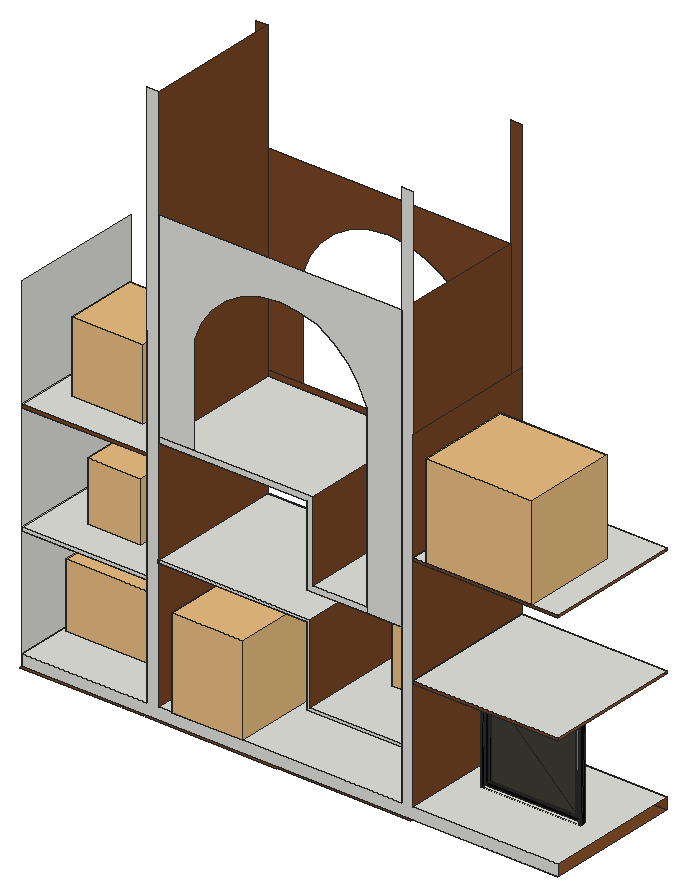
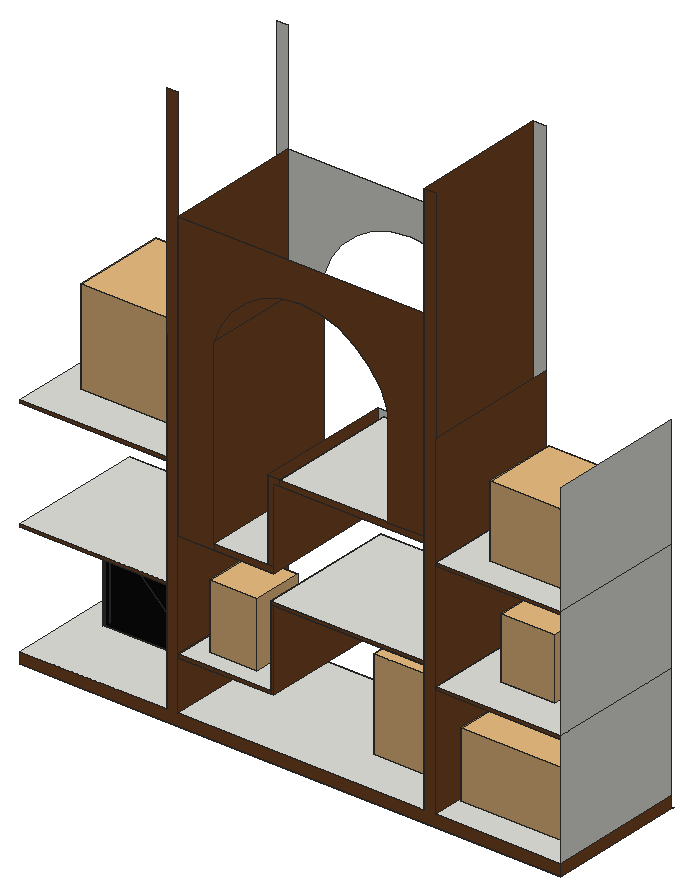
# SketchUp Ruby script. Lengths in inches.
U = 1.inch
M = Sketchup.active_model
def pt(a) = Geom::Point3d.new(a.map { |v| v * U })
def face(e, loops, mat)
  f = e.add_face(loops[0].map { |a| pt(a) })
  loops[1..].each { |l| e.add_face(l.map { |a| pt(a) }).erase! }
  f.material = f.back_material = mat if mat
  f
end
# faces: each face lists its corners as indices into pts; further lists are holes
def faces(e, pts, list, mat = nil) = list.each { |f| face(e, (f[0].is_a?(Array) ? f : [f]).map { |l| l.map { |i| pts[i] } }, mat) }
# xy, xz, yz: faces in a plane at the given z, y or x. An outline is a flat list of corners, or four numbers for a rectangle; further outlines are holes
def ring(l) = l.size == 4 ? [[l[0], l[1]], [l[2], l[1]], [l[2], l[3]], [l[0], l[3]]] : l.each_slice(2).to_a
def flat(e, list, mat, &to3) = list.each { |f| face(e, (f[0].is_a?(Array) ? f : [f]).map { |l| ring(l).map { |u, v| to3.(u, v) } }, mat) }
def xy(e, z, list, mat = nil) = flat(e, list, mat) { |x, y| [x, y, z] }
def xz(e, y, list, mat = nil) = flat(e, list, mat) { |x, z| [x, y, z] }
def yz(e, x, list, mat = nil) = flat(e, list, mat) { |y, z| [x, y, z] }
def lines(e, pts, list) = list.each { |a, b| e.add_line(pt(pts[a]), pt(pts[b])) }
# prism: a flat outline (further loops are holes) pulled along v
def prism(e, loops, v, mat = nil)
  f = face(e, loops, mat); d = Geom::Vector3d.new(v.map { |x| x * U })
  f.pushpull(f.normal.samedirection?(d) ? d.length : -d.length)
end
def box(e, o, s, mat = nil) = prism(e, [[o, [o[0] + s[0], o[1], o[2]], [o[0] + s[0], o[1] + s[1], o[2]], [o[0], o[1] + s[1], o[2]]]], [0, 0, s[2]], mat)
def at(x, y, z, deg = 0) = Geom::Transformation.translation(pt([x, y, z])) * Geom::Transformation.rotation(ORIGIN, Z_AXIS, deg.degrees)
def axes(o, x, y, z) = Geom::Transformation.new([*x, 0, *y, 0, *z, 0, *pt(o).to_a, 1])
def part(name) = M.definitions.add(name)
# library, detail: a bought-in or finely detailed component or shape, given as its bounding box
def library(name, o, s) = part(name).tap { |d| box(d.entities, o, s) }
def detail(e, o, s) = box(e.add_group.entities, o, s)
def put(e, d, t, mat = nil) = e.add_instance(d, t).tap { |i| i.material = mat if mat }
def group(e, t, mat = nil) = e.add_group.tap { |g| g.transformation = t; g.material = mat if mat }.entities
root = M.entities
M.materials.add("Material~12").color = [12, 12, 12]
M.materials.add("Material~27").color = [10, 10, 10]
M.materials.add("Material~28").color = [156, 145, 125]
M.materials.add("Material~29").color = [62, 62, 54]
M.materials.add("[Wood Veneer 01]").color = [120, 70, 37]
c1 = library("Group3\#1",[-226.43,63.68,0],[21.09,21.08,29.58])
c2 = library("Group145\#1",[5.875,6.46,9.56],[20.8,10.13,11.36])
c3 = library("Potted Plant",[38.42,1.35,0],[44.68,49.99,41.74])
c4 = library("Pot Nice",[-24.73,-24.73,-0.79],[49.46,49.46,53.07])
c5 = library("Desktop globe",[0,0,0],[12.93,11.94,21.27])
c6 = library("PLANTS",[8.46,16.75,1.64],[23.16,16.42,22.13])
c7 = part("3DGeom~7_Defintion")
xy(c7.entities,14.63,[[-469.76,-662.07,-453.03,-645.34,-469.55,277.5],[-469.76,-662.07,513.32,-645.34,-453.03,-645.34],[-469.76,-662.07,530.04,-662.07,513.32,-645.34],[530.04,-662.07,513.52,260.77,513.32,-645.34],[530.04,-662.07,530.24,277.5,513.52,260.77],
  [-453.03,-645.34,-452.83,260.77,-469.55,277.5],[-452.83,260.77,530.24,277.5,-469.55,277.5],[-452.83,260.77,513.52,260.77,530.24,277.5]])
xz(c7.entities,-645.34,[[-453.03,2.4375,-453.03,14.63,513.32,2.4375],[513.32,2.4375,-453.03,14.63,513.32,14.63]])
xz(c7.entities,260.77,[[-452.83,2.4375,513.52,14.63,-452.83,14.63],[-452.83,2.4375,513.52,2.4375,513.52,14.63]])
p = [[-452.83,260.77,14.63],[-453.03,-645.34,14.63],[-453.03,-645.34,2.4375],[-452.83,260.77,2.4375],[513.32,-645.34,14.63],[513.52,260.77,14.63],
  [513.52,260.77,2.4375],[513.32,-645.34,2.4375]]
faces(c7.entities,p,[[0,1,2],[2,3,0],[4,5,6],[6,7,4]])
c8 = part("Group74\#2")
put(c8.entities,c7,axes([-1.26,-0.81,45.42],[0.01556,0,0],[0,0,0.01556],[0,-0.0137,0]),"Material~27")
c9 = part("Group73\#2")
put(c9.entities,c8,at(0,0,0))
c10 = part("3DGeom~8_Defintion")
xy(c10.entities,0,[[-469.76,-662.07,-469.55,277.5,530.04,-662.07],[530.04,-662.07,-469.55,277.5,530.24,277.5]],"Material~28")
xz(c10.entities,-662.07,[[-469.76,0,530.04,0,530.04,14.63],[-469.76,0,530.04,14.63,-469.76,14.63]],"Material~28")
xz(c10.entities,277.5,[[-469.55,0,-469.55,14.63,530.24,0],[530.24,0,-469.55,14.63,530.24,14.63]],"Material~28")
p = [[-469.55,277.5,0],[-469.76,-662.07,0],[-469.76,-662.07,14.63],[-469.55,277.5,14.63],[530.04,-662.07,0],[530.24,277.5,0],
  [530.24,277.5,14.63],[530.04,-662.07,14.63]]
faces(c10.entities,p,[[0,1,2],[2,3,0],[4,5,6],[6,7,4]],"Material~28")
c11 = part("Group76\#2")
put(c11.entities,c10,axes([-1.26,-0.81,45.42],[0.01556,0,0],[0,0,0.01556],[0,-0.0137,0]),"Material~28")
c12 = part("Group75\#2")
put(c12.entities,c11,at(0,0,0))
c13 = part("3DGeom~13_Defintion")
xy(c13.entities,2.52,[[-468.71,-667.68,531.09,-667.68,-468.5,269.8],[531.09,-667.68,531.29,269.8,-468.5,269.8]],"Material~29")
c14 = part("Group86\#2")
put(c14.entities,c13,axes([-1.26,-0.81,45.42],[0.01504,0,0],[0,0,0.01504],[0,-0.01324,0]),"Material~29")
c15 = part("Group85\#2")
put(c15.entities,c14,at(0,0,0))
c16 = part("3DGeom~10_Defintion")
xy(c16.entities,58.03,[[-471.35,-6.46,515.55,6.46,-458.43,6.46],[-471.35,-6.46,528.47,-6.46,515.55,6.46],[-458.25,916.93,515.73,916.93,-471.17,929.85],[515.73,916.93,528.65,929.85,-471.17,929.85]],"Material~28")
c17 = part("Group80\#2")
put(c17.entities,c16,axes([-1.26,-0.65,34.26],[0.01762,0,0],[0,0,0.01762],[0,-0.01552,0]),"Material~28")
c18 = part("Group79\#2")
put(c18.entities,c17,at(0,0,0))
c19 = part("3DGeom~11_Defintion")
xy(c19.entities,0,[[-471.35,-6.46,-458.43,6.46,515.55,6.46],[-471.35,-6.46,515.55,6.46,528.47,-6.46],[-458.25,916.93,-471.17,929.85,515.73,916.93],[515.73,916.93,-471.17,929.85,528.65,929.85]])
xz(c19.entities,-6.46,[[-471.35,0,528.47,0,528.47,58.03],[-471.35,0,528.47,58.03,-471.35,58.03]])
xz(c19.entities,6.46,[[-458.43,0,-458.43,58.03,515.55,0],[515.55,0,-458.43,58.03,515.55,58.03]])
xz(c19.entities,916.93,[[-458.25,0,515.73,0,-458.25,58.03],[515.73,0,515.73,58.03,-458.25,58.03]])
xz(c19.entities,929.85,[[-471.17,0,-471.17,58.03,528.65,58.03],[-471.17,0,528.65,58.03,528.65,0]])
p = [[-458.43,6.46,0],[-471.35,-6.46,0],[-471.35,-6.46,58.03],[-458.43,6.46,58.03],[528.47,-6.46,0],[515.55,6.46,0],
  [515.55,6.46,58.03],[528.47,-6.46,58.03],[-458.25,916.93,0],[-458.25,916.93,58.03],[-471.17,929.85,58.03],[-471.17,929.85,0],
  [528.65,929.85,0],[528.65,929.85,58.03],[515.73,916.93,58.03],[515.73,916.93,0]]
faces(c19.entities,p,[[0,1,2],[2,3,0],[4,5,6],[6,7,4],[8,9,10],[10,11,8],[12,13,14],[14,15,12]])
c20 = part("Group82\#2")
put(c20.entities,c19,axes([-1.26,-0.65,34.26],[0.01762,0,0],[0,0,0.01762],[0,-0.01552,0]),"Material~27")
c21 = part("Group81\#2")
put(c21.entities,c20,at(0,0,0))
c22 = part("3DGeom~6_Defintion")
xy(c22.entities,0,[[-470.59,-643.09,-470.4,291.53,529.41,291.53],[-470.59,-643.09,529.41,291.53,529.22,-643.09]])
xy(c22.entities,11.05,[[-470.59,-643.09,529.22,-643.09,529.41,291.53],[-470.59,-643.09,529.41,291.53,-470.4,291.53]])
xz(c22.entities,-643.09,[[-470.59,0,529.22,0,529.22,11.05],[-470.59,0,529.22,11.05,-470.59,11.05]])
xz(c22.entities,291.53,[[-470.4,0,-470.4,11.05,529.41,0],[529.41,0,-470.4,11.05,529.41,11.05]])
p = [[-470.4,291.53,0],[-470.59,-643.09,0],[-470.59,-643.09,11.05],[-470.4,291.53,11.05],[529.22,-643.09,0],[529.41,291.53,0],
  [529.41,291.53,11.05],[529.22,-643.09,11.05]]
faces(c22.entities,p,[[0,1,2],[2,3,0],[4,5,6],[6,7,4]])
c23 = part("Group72\#2")
put(c23.entities,c22,axes([-1.26,-0.65,45.42],[0.01717,0,0],[0,0,0.01717],[0,-0.01512,0]),"Material~12")
c24 = part("Group71\#2")
put(c24.entities,c23,at(0,0,0))
c25 = part("3DGeom~9_Defintion")
xy(c25.entities,58.03,[[373.52,427.46,360.6,440.375,-562.79,427.64],[-562.79,427.64,360.6,440.375,-549.87,440.56],[360.6,1414.36,-562.79,1427.46,-549.87,1414.54],[360.6,1414.36,373.52,1427.28,-562.79,1427.46]],"Material~28")
c26 = part("Group78\#2")
put(c26.entities,c25,axes([-17.1,-0.65,40.73],[0,0,-0.01762],[0.01762,0,0],[0,-0.01552,0]),"Material~28")
c27 = part("Group77\#2")
put(c27.entities,c26,at(0,0,0))
c28 = part("3DGeom~12_Defintion")
xy(c28.entities,0,[[373.52,427.46,-562.79,427.64,360.6,440.375],[-562.79,427.64,-549.87,440.56,360.6,440.375],[360.6,1414.36,-549.87,1414.54,-562.79,1427.46],[360.6,1414.36,-562.79,1427.46,373.52,1427.28]])
p = [[-562.79,427.64,0],[373.52,427.46,0],[373.52,427.46,58.03],[-562.79,427.64,58.03],[373.52,427.46,0],[360.6,440.375,0],
  [360.6,440.375,58.03],[373.52,427.46,58.03],[-549.87,440.56,0],[-562.79,427.64,0],[-562.79,427.64,58.03],[-549.87,440.56,58.03],
  [360.6,440.375,0],[-549.87,440.56,0],[-549.87,440.56,58.03],[360.6,440.375,58.03],[360.6,1414.36,0],[360.6,1414.36,58.03],
  [-549.87,1414.54,58.03],[-549.87,1414.54,0],[373.52,1427.28,0],[373.52,1427.28,58.03],[360.6,1414.36,58.03],[360.6,1414.36,0],
  [-549.87,1414.54,0],[-549.87,1414.54,58.03],[-562.79,1427.46,58.03],[-562.79,1427.46,0],[-562.79,1427.46,0],[-562.79,1427.46,58.03],
  [373.52,1427.28,58.03],[373.52,1427.28,0]]
faces(c28.entities,p,[[0,1,2],[2,3,0],[4,5,6],[6,7,4],[8,9,10],[10,11,8],[12,13,14],[14,15,12],
  [16,17,18],[18,19,16],[20,21,22],[22,23,20],[24,25,26],[26,27,24],[28,29,30],[30,31,28]])
c29 = part("Group84\#2")
put(c29.entities,c28,axes([-17.1,-0.65,40.73],[0,0,-0.01762],[0.01762,0,0],[0,-0.01552,0]),"Material~27")
c30 = part("Group83\#2")
put(c30.entities,c29,at(0,0,0))
xy(root,37.59,[[12.38,2,30.26,2.47],[30.5,2,34.26,2.47],[34.5,2,57.76,2.47],[58,2,81.38,2.47],[12.38,2.47,81.38,26.47],
  [81.38,2.47,106.84,26.47]],"[Wood Veneer 01]")
xy(root,39.59,[[12.38,2.47,34.34,26.47],[36.46,2.47,79.29,26.47],[81.29,2.47,106.84,26.47]])
xy(root,48.32,[[62.64,2.47,79.29,26.47]])
xy(root,48.82,[[63.14,2.47,79.29,26.47]])
xy(root,59.02,[[12.38,2.47,34.34,26.47]])
xy(root,59.02,[[81.29,2.47,106.84,26.47]],"[Wood Veneer 01]")
xy(root,59.52,[[12.38,2.47,34.34,26.47],[81.29,2.47,106.84,26.47]])
xy(root,62.32,[[36.38,2.47,62.64,26.47]])
xy(root,62.82,[[36.38,2.47,63.14,26.47]])
xy(root,67.32,[[62.64,2.47,79.29,26.47]])
xy(root,68.32,[[63.64,2.47,73.11,26.47]])
xy(root,78.45,[[12.38,2.47,34.34,26.47]])
xy(root,78.45,[[81.29,2.47,106.84,26.47]],"[Wood Veneer 01]")
xy(root,78.95,[[12.38,2.47,34.34,26.47],[81.29,2.47,106.84,26.47]])
xy(root,81.32,[[36.38,2.47,62.64,26.47]])
xz(root,2.47,[[12.38,37.59,106.84,37.59,106.84,39.59,81.29,39.59,81.29,136.75,79.29,136.75,79.29,39.59,36.46,39.59,36.46,62.32,36.38,62.32,36.38,62.82,36.46,62.82,36.46,82.32,36.38,82.32,36.38,117.82,36.46,117.82,36.46,136.75,34.34,136.75,34.34,39.59,12.38,39.59],[62.64,48.32,79.29,48.32,79.29,48.82,63.14,48.82,63.14,62.82,36.46,62.82,36.46,62.32,62.64,62.32],[12.38,59.02,34.34,59.52],[62.64,67.32,73.11,67.32,73.11,68.32,63.64,68.32,63.64,82.32,36.46,82.32,36.46,81.32,62.64,81.32],[73.11,67.32,79.29,67.32,79.29,117.32,36.46,117.32,36.46,82.32,42.64,82.32,42.64,99.82,43.96,102.9375,45.9,105.7,48.38,108,51.3,109.72,54.51,110.78,57.875,111.14,61.24,110.78,64.45,109.72,67.36,108,69.85,105.7,71.79,102.9375,73.11,99.82]])
xz(root,2.47,[[81.29,59.02,106.84,59.52],[36.38,62.32,36.46,62.82],[12.38,78.45,34.34,78.95],[81.29,78.45,106.84,78.95]],"[Wood Veneer 01]")
xz(root,26.47,[[12.38,37.59,12.38,39.59,34.34,39.59,34.34,136.75,36.46,136.75,36.46,117.82,36.38,117.82,36.38,81.32,36.46,81.32,36.46,62.82,36.38,62.82,36.38,62.32,36.46,62.32,36.46,39.59,79.29,39.59,79.29,136.75,81.29,136.75,81.29,39.59,106.84,39.59,106.84,37.59],[62.64,48.32,63.14,49.32],[63.14,48.32,73.11,48.82],[73.11,48.32,79.29,48.82],[62.64,49.32,63.14,62.32],
  [12.38,59.02,34.34,59.52],[81.29,59.02,106.84,59.52],[36.38,62.32,36.46,62.82],[36.46,62.32,61.64,62.82],[61.64,62.32,63.14,62.82],
  [73.11,67.32,73.11,99.82,71.79,102.9375,69.85,105.7,67.36,108,64.45,109.72,61.24,110.78,57.875,111.14,54.51,110.78,51.3,109.72,48.38,108,45.9,105.7,43.96,102.9375,42.64,99.82,42.64,82.32,36.46,82.32,36.46,117.32,79.29,117.32,79.29,67.32],[62.64,67.32,73.11,68.32],[62.64,68.32,62.64,81.32,61.64,81.32,61.64,82.32,63.64,82.32,63.64,68.32],[12.38,78.45,34.34,78.95],[81.29,78.45,106.84,78.95],
  [36.38,81.32,36.46,82.32],[36.46,81.32,61.64,82.32]],"[Wood Veneer 01]")
yz(root,12.38,[[2.47,39.59,26.47,59.52],[2.47,59.52,26.47,78.95],[2.47,78.95,26.47,98.39]])
yz(root,12.38,[[2.47,37.59,26.47,39.59]],"[Wood Veneer 01]")
yz(root,34.34,[[2.47,39.59,26.47,59.52],[2.47,59.52,26.47,78.95],[2.47,78.95,26.47,98.39]],"[Wood Veneer 01]")
yz(root,36.38,[[2.47,62.32,26.47,62.82]],"[Wood Veneer 01]")
yz(root,36.46,[[2.47,39.59,26.47,136.75]],"[Wood Veneer 01]")
yz(root,62.64,[[2.47,48.32,26.47,62.32],[2.47,67.32,26.47,81.32]],"[Wood Veneer 01]")
yz(root,63.14,[[2.47,48.82,26.47,62.82]],"[Wood Veneer 01]")
yz(root,63.64,[[2.47,68.32,26.47,82.32]],"[Wood Veneer 01]")
yz(root,73.11,[[2.47,68.32,26.47,99.82]],"[Wood Veneer 01]")
yz(root,79.29,[[2.47,39.59,26.47,48.32],[2.47,48.32,26.47,48.82],[2.47,48.82,26.47,67.32],[2.47,67.32,26.47,117.32]],"[Wood Veneer 01]")
yz(root,81.29,[[2.47,39.59,26.47,59.52],[2.47,59.52,26.47,78.95],[2.47,78.95,26.47,98.39]],"[Wood Veneer 01]")
put(root,c1,axes([151.65,-29.88,78.95],[0.59809,0,0],[0,0.6048,0],[0,0,0.42]))
put(root,c2,at(7.3,4.77,30.01))
put(root,c3,axes([10.89,8.53,59.52],[0.2097,0,0],[0,0.21818,0],[0,0,0.25242]))
put(root,c4,axes([45.07,10.57,39.82],[0.25357,0,0],[0,0.3276,0],[0,0,0.2964]))
put(root,c5,axes([68.01,14.47,48.82],[0.64,0,0],[0,0.74,0],[0,0,0.53]))
put(root,c6,axes([76.72,-14.28,77.74],[0.81,0,0],[0,1,0],[0,0,0.74]))
put(root,c9,at(94.52,14.34,5.21))
put(root,c12,at(94.52,14.34,5.21))
put(root,c15,at(94.52,14.34,5.21))
put(root,c18,at(94.52,14.34,5.21))
put(root,c21,at(94.52,14.34,5.21))
put(root,c24,at(94.52,14.34,5.21))
put(root,c27,at(94.52,14.34,5.21))
put(root,c30,at(94.52,14.34,5.21))
